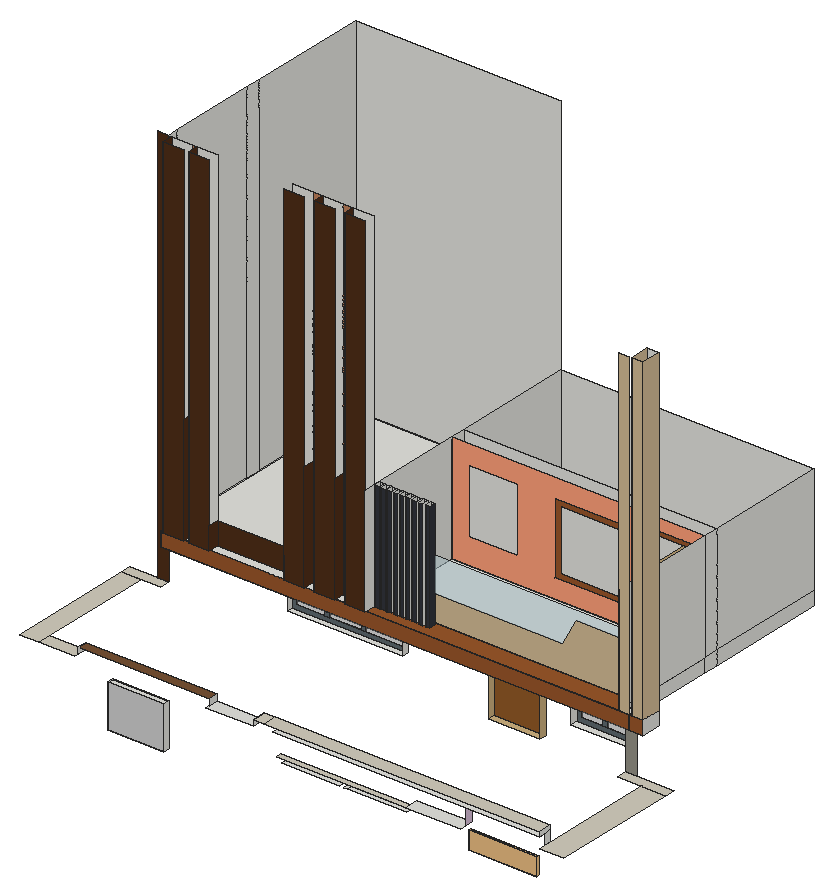
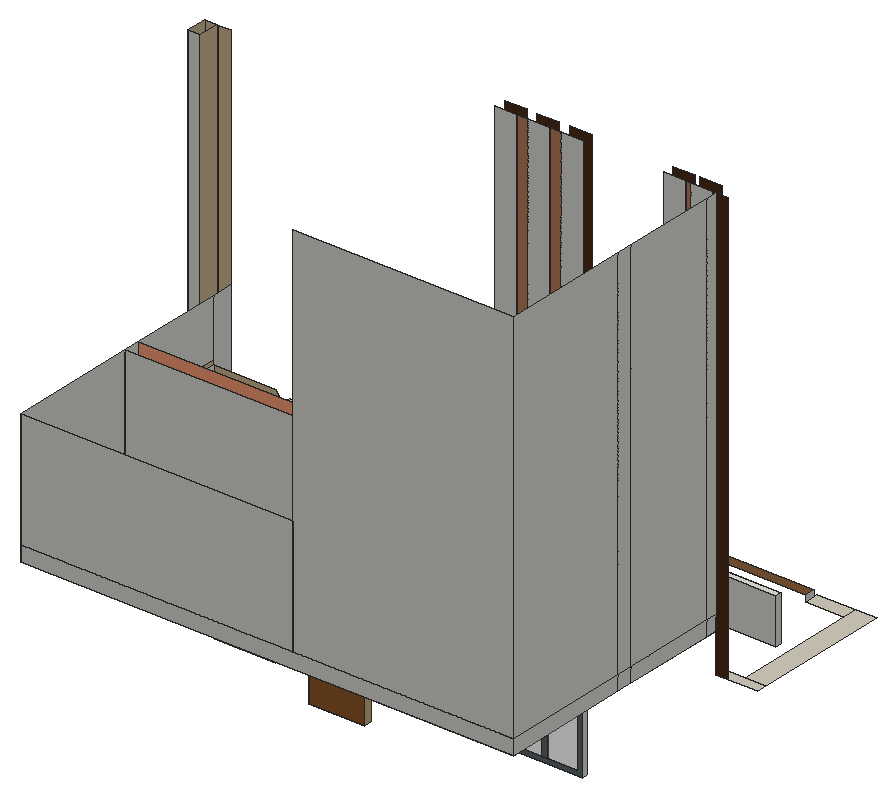
# SketchUp Ruby script. Lengths in inches.
U = 1.inch
M = Sketchup.active_model
def pt(a) = Geom::Point3d.new(a.map { |v| v * U })
def face(e, loops, mat)
  f = e.add_face(loops[0].map { |a| pt(a) })
  loops[1..].each { |l| e.add_face(l.map { |a| pt(a) }).erase! }
  f.material = f.back_material = mat if mat
  f
end
# faces: each face lists its corners as indices into pts; further lists are holes
def faces(e, pts, list, mat = nil) = list.each { |f| face(e, (f[0].is_a?(Array) ? f : [f]).map { |l| l.map { |i| pts[i] } }, mat) }
# xy, xz, yz: faces in a plane at the given z, y or x. An outline is a flat list of corners, or four numbers for a rectangle; further outlines are holes
def ring(l) = l.size == 4 ? [[l[0], l[1]], [l[2], l[1]], [l[2], l[3]], [l[0], l[3]]] : l.each_slice(2).to_a
def flat(e, list, mat, &to3) = list.each { |f| face(e, (f[0].is_a?(Array) ? f : [f]).map { |l| ring(l).map { |u, v| to3.(u, v) } }, mat) }
def xy(e, z, list, mat = nil) = flat(e, list, mat) { |x, y| [x, y, z] }
def xz(e, y, list, mat = nil) = flat(e, list, mat) { |x, z| [x, y, z] }
def yz(e, x, list, mat = nil) = flat(e, list, mat) { |y, z| [x, y, z] }
def lines(e, pts, list) = list.each { |a, b| e.add_line(pt(pts[a]), pt(pts[b])) }
# prism: a flat outline (further loops are holes) pulled along v
def prism(e, loops, v, mat = nil)
  f = face(e, loops, mat); d = Geom::Vector3d.new(v.map { |x| x * U })
  f.pushpull(f.normal.samedirection?(d) ? d.length : -d.length)
end
def box(e, o, s, mat = nil) = prism(e, [[o, [o[0] + s[0], o[1], o[2]], [o[0] + s[0], o[1] + s[1], o[2]], [o[0], o[1] + s[1], o[2]]]], [0, 0, s[2]], mat)
def at(x, y, z, deg = 0) = Geom::Transformation.translation(pt([x, y, z])) * Geom::Transformation.rotation(ORIGIN, Z_AXIS, deg.degrees)
def axes(o, x, y, z) = Geom::Transformation.new([*x, 0, *y, 0, *z, 0, *pt(o).to_a, 1])
def part(name) = M.definitions.add(name)
# library, detail: a bought-in or finely detailed component or shape, given as its bounding box
def library(name, o, s) = part(name).tap { |d| box(d.entities, o, s) }
def detail(e, o, s) = box(e.add_group.entities, o, s)
def put(e, d, t, mat = nil) = e.add_instance(d, t).tap { |i| i.material = mat if mat }
def group(e, t, mat = nil) = e.add_group.tap { |g| g.transformation = t; g.material = mat if mat }.entities
root = M.entities
M.materials.add("[0026_LightSalmon]").color = [255, 160, 122]
M.materials.add("[0046_Gold]").color = [226, 191, 0]
M.materials.add("[0118_Thistle]").color = [216, 191, 216]
M.materials.add("[Carrera Marble]").color = [207, 207, 207]
M.materials.add("[Formica Beige]").color = [211, 187, 149]
M.materials.add("[Formica Graystone]").color = [209, 204, 189]
M.materials.add("[Formica Graystone]1").color = [149, 146, 135]
M.materials.add("[Formica Laminate Dark]").color = [50, 53, 60]
M.materials.add("[Formica Speckled Grey]").color = [94, 105, 111]
M.materials.add("[Sandstone]").color = [118, 81, 52]
M.materials.add("[Translucent Glass Gray]").color = [128, 128, 128]
M.materials["[Translucent Glass Gray]"].alpha = 0.5
M.materials.add("[Translucent Glass Safety]").color = [204, 235, 244]
M.materials["[Translucent Glass Safety]"].alpha = 0.5
M.materials.add("[Wood Cherry Original]").color = [152, 86, 42]
M.materials.add("[Wood Floor Light]").color = [204, 176, 127]
M.materials.add("[Wood Floor Parquet]").color = [145, 89, 39]
M.materials.add("[Wood Veneer 01]").color = [79, 46, 24]
M.materials.add("[Wood Veneer 02]").color = [190, 128, 91]
c1 = library("Shloka",[1.82,0,0],[112.97,25.6,12])
xy(root,17.66,[[410.04,348.07,486.1,358.26]],"[Wood Floor Light]")
xy(root,51.82,[[530.86,348.07,613.92,359.32]])
xy(root,56.31,[[116.08,348.07,284.86,355.95]])
xy(root,58.17,[[130.9,0,212.59,8.25]])
xy(root,96.37,[[[377.34,9.54,462.5,17.41],[458.64,12.51,458.96,12.55,459.26,12.67,459.52,12.875,459.72,13.13,459.85,13.43,459.89,13.76,459.85,14.08,459.72,14.38,459.52,14.64,459.26,14.84,458.96,14.96,458.64,15.01,458.32,14.96,458.01,14.84,457.76,14.64,457.56,14.38,457.43,14.08,457.39,13.76,457.43,13.43,457.56,13.13,457.76,12.875,458.01,12.67,458.32,12.55],[453.95,12.51,454.28,12.55,454.58,12.67,454.84,12.875,455.03,13.13,455.16,13.43,455.2,13.76,455.16,14.08,455.03,14.38,454.84,14.64,454.58,14.84,454.28,14.96,453.95,15.01,453.63,14.96,453.33,14.84,453.07,14.64,452.87,14.38,452.74,14.08,452.7,13.76,452.74,13.43,452.87,13.13,453.07,12.875,453.33,12.67,453.63,12.55],[448.45,12.51,448.78,12.55,449.08,12.67,449.34,12.875,449.53,13.13,449.66,13.43,449.7,13.76,449.66,14.08,449.53,14.38,449.34,14.64,449.08,14.84,448.78,14.96,448.45,15.01,448.13,14.96,447.83,14.84,447.57,14.64,447.37,14.38,447.24,14.08,447.2,13.76,447.24,13.43,447.37,13.13,447.57,12.875,447.83,12.67,448.13,12.55],[442.45,12.51,442.78,12.55,443.08,12.67,443.34,12.875,443.53,13.13,443.66,13.43,443.7,13.76,443.66,14.08,443.53,14.38,443.34,14.64,443.08,14.84,442.78,14.96,442.45,15.01,442.13,14.96,441.83,14.84,441.57,14.64,441.37,14.38,441.24,14.08,441.2,13.76,441.24,13.43,441.37,13.13,441.57,12.875,441.83,12.67,442.13,12.55],[436.2,12.51,436.53,12.55,436.83,12.67,437.09,12.875,437.28,13.13,437.41,13.43,437.45,13.76,437.41,14.08,437.28,14.38,437.09,14.64,436.83,14.84,436.53,14.96,436.2,15.01,435.88,14.96,435.58,14.84,435.32,14.64,435.12,14.38,434.99,14.08,434.95,13.76,434.99,13.43,435.12,13.13,435.32,12.875,435.58,12.67,435.88,12.55],[430.51,12.51,430.84,12.55,431.14,12.67,431.4,12.875,431.6,13.13,431.72,13.43,431.76,13.76,431.72,14.08,431.6,14.38,431.4,14.64,431.14,14.84,430.84,14.96,430.51,15.01,430.19,14.96,429.89,14.84,429.63,14.64,429.43,14.38,429.31,14.08,429.26,13.76,429.31,13.43,429.43,13.13,429.63,12.875,429.89,12.67,430.19,12.55],[424.64,12.51,424.96,12.55,425.26,12.67,425.52,12.875,425.72,13.13,425.85,13.43,425.89,13.76,425.85,14.08,425.72,14.38,425.52,14.64,425.26,14.84,424.96,14.96,424.64,15.01,424.32,14.96,424.01,14.84,423.76,14.64,423.56,14.38,423.43,14.08,423.39,13.76,423.43,13.43,423.56,13.13,423.76,12.875,424.01,12.67,424.32,12.55],[418.89,12.51,419.21,12.55,419.51,12.67,419.77,12.875,419.97,13.13,420.1,13.43,420.14,13.76,420.1,14.08,419.97,14.38,419.77,14.64,419.51,14.84,419.21,14.96,418.89,15.01,418.57,14.96,418.26,14.84,418.01,14.64,417.81,14.38,417.68,14.08,417.64,13.76,417.68,13.43,417.81,13.13,418.01,12.875,418.26,12.67,418.57,12.55],[414.01,12.51,414.34,12.55,414.64,12.67,414.9,12.875,415.1,13.13,415.22,13.43,415.26,13.76,415.22,14.08,415.1,14.38,414.9,14.64,414.64,14.84,414.34,14.96,414.01,15.01,413.69,14.96,413.39,14.84,413.13,14.64,412.93,14.38,412.81,14.08,412.76,13.76,412.81,13.43,412.93,13.13,413.13,12.875,413.39,12.67,413.69,12.55],[408.45,12.51,408.78,12.55,409.08,12.67,409.34,12.875,409.53,13.13,409.66,13.43,409.7,13.76,409.66,14.08,409.53,14.38,409.34,14.64,409.08,14.84,408.78,14.96,408.45,15.01,408.13,14.96,407.83,14.84,407.57,14.64,407.37,14.38,407.24,14.08,407.2,13.76,407.24,13.43,407.37,13.13,407.57,12.875,407.83,12.67,408.13,12.55],[402.58,12.51,402.9,12.55,403.2,12.67,403.46,12.875,403.66,13.13,403.78,13.43,403.83,13.76,403.78,14.08,403.66,14.38,403.46,14.64,403.2,14.84,402.9,14.96,402.58,15.01,402.25,14.96,401.95,14.84,401.69,14.64,401.49,14.38,401.37,14.08,401.33,13.76,401.37,13.43,401.49,13.13,401.69,12.875,401.95,12.67,402.25,12.55],[396.95,12.51,397.28,12.55,397.58,12.67,397.84,12.875,398.03,13.13,398.16,13.43,398.2,13.76,398.16,14.08,398.03,14.38,397.84,14.64,397.58,14.84,397.28,14.96,396.95,15.01,396.63,14.96,396.33,14.84,396.07,14.64,395.87,14.38,395.74,14.08,395.7,13.76,395.74,13.43,395.87,13.13,396.07,12.875,396.33,12.67,396.63,12.55],[390.45,12.51,390.78,12.55,391.08,12.67,391.34,12.875,391.53,13.13,391.66,13.43,391.7,13.76,391.66,14.08,391.53,14.38,391.34,14.64,391.08,14.84,390.78,14.96,390.45,15.01,390.13,14.96,389.83,14.84,389.57,14.64,389.37,14.38,389.24,14.08,389.2,13.76,389.24,13.43,389.37,13.13,389.57,12.875,389.83,12.67,390.13,12.55],[384.7,12.51,385.03,12.55,385.33,12.67,385.59,12.875,385.78,13.13,385.91,13.43,385.95,13.76,385.91,14.08,385.78,14.38,385.59,14.64,385.33,14.84,385.03,14.96,384.7,15.01,384.38,14.96,384.08,14.84,383.82,14.64,383.62,14.38,383.49,14.08,383.45,13.76,383.49,13.43,383.62,13.13,383.82,12.875,384.08,12.67,384.38,12.55],[380.14,12.51,380.47,12.55,380.77,12.67,381.03,12.875,381.23,13.13,381.35,13.43,381.39,13.76,381.35,14.08,381.23,14.38,381.03,14.64,380.77,14.84,380.47,14.96,380.14,15.01,379.82,14.96,379.52,14.84,379.26,14.64,379.06,14.38,378.94,14.08,378.89,13.76,378.94,13.43,379.06,13.13,379.26,12.875,379.52,12.67,379.82,12.55]],[468.46,9.54,474.42,17.41],[[474.42,9.54,560.77,17.41],[555.89,12.51,556.21,12.55,556.51,12.67,556.77,12.875,556.97,13.13,557.1,13.43,557.14,13.76,557.1,14.08,556.97,14.38,556.77,14.64,556.51,14.84,556.21,14.96,555.89,15.01,555.57,14.96,555.26,14.84,555.01,14.64,554.81,14.38,554.68,14.08,554.64,13.76,554.68,13.43,554.81,13.13,555.01,12.875,555.26,12.67,555.57,12.55],[550.39,12.51,550.71,12.55,551.01,12.67,551.27,12.875,551.47,13.13,551.6,13.43,551.64,13.76,551.6,14.08,551.47,14.38,551.27,14.64,551.01,14.84,550.71,14.96,550.39,15.01,550.07,14.96,549.76,14.84,549.51,14.64,549.31,14.38,549.18,14.08,549.14,13.76,549.18,13.43,549.31,13.13,549.51,12.875,549.76,12.67,550.07,12.55],[544.76,12.51,545.09,12.55,545.39,12.67,545.65,12.875,545.85,13.13,545.97,13.43,546.01,13.76,545.97,14.08,545.85,14.38,545.65,14.64,545.39,14.84,545.09,14.96,544.76,15.01,544.44,14.96,544.14,14.84,543.88,14.64,543.68,14.38,543.56,14.08,543.51,13.76,543.56,13.43,543.68,13.13,543.88,12.875,544.14,12.67,544.44,12.55],[539.51,12.51,539.84,12.55,540.14,12.67,540.4,12.875,540.6,13.13,540.72,13.43,540.76,13.76,540.72,14.08,540.6,14.38,540.4,14.64,540.14,14.84,539.84,14.96,539.51,15.01,539.19,14.96,538.89,14.84,538.63,14.64,538.43,14.38,538.31,14.08,538.26,13.76,538.31,13.43,538.43,13.13,538.63,12.875,538.89,12.67,539.19,12.55],[533.7,12.51,534.03,12.55,534.33,12.67,534.59,12.875,534.78,13.13,534.91,13.43,534.95,13.76,534.91,14.08,534.78,14.38,534.59,14.64,534.33,14.84,534.03,14.96,533.7,15.01,533.38,14.96,533.08,14.84,532.82,14.64,532.62,14.38,532.49,14.08,532.45,13.76,532.49,13.43,532.62,13.13,532.82,12.875,533.08,12.67,533.38,12.55],[528.2,12.51,528.53,12.55,528.83,12.67,529.09,12.875,529.28,13.13,529.41,13.43,529.45,13.76,529.41,14.08,529.28,14.38,529.09,14.64,528.83,14.84,528.53,14.96,528.2,15.01,527.88,14.96,527.58,14.84,527.32,14.64,527.12,14.38,526.99,14.08,526.95,13.76,526.99,13.43,527.12,13.13,527.32,12.875,527.58,12.67,527.88,12.55],[522.33,12.51,522.65,12.55,522.95,12.67,523.21,12.875,523.41,13.13,523.53,13.43,523.58,13.76,523.53,14.08,523.41,14.38,523.21,14.64,522.95,14.84,522.65,14.96,522.33,15.01,522,14.96,521.7,14.84,521.44,14.64,521.24,14.38,521.12,14.08,521.08,13.76,521.12,13.43,521.24,13.13,521.44,12.875,521.7,12.67,522,12.55],[517.01,12.51,517.34,12.55,517.64,12.67,517.9,12.875,518.1,13.13,518.22,13.43,518.26,13.76,518.22,14.08,518.1,14.38,517.9,14.64,517.64,14.84,517.34,14.96,517.01,15.01,516.69,14.96,516.39,14.84,516.13,14.64,515.93,14.38,515.81,14.08,515.76,13.76,515.81,13.43,515.93,13.13,516.13,12.875,516.39,12.67,516.69,12.55],[511.7,12.51,512.03,12.55,512.33,12.67,512.59,12.875,512.78,13.13,512.91,13.43,512.95,13.76,512.91,14.08,512.78,14.38,512.59,14.64,512.33,14.84,512.03,14.96,511.7,15.01,511.38,14.96,511.08,14.84,510.82,14.64,510.62,14.38,510.49,14.08,510.45,13.76,510.49,13.43,510.62,13.13,510.82,12.875,511.08,12.67,511.38,12.55],[506.08,12.51,506.4,12.55,506.7,12.67,506.96,12.875,507.16,13.13,507.28,13.43,507.33,13.76,507.28,14.08,507.16,14.38,506.96,14.64,506.7,14.84,506.4,14.96,506.08,15.01,505.75,14.96,505.45,14.84,505.19,14.64,504.99,14.38,504.87,14.08,504.83,13.76,504.87,13.43,504.99,13.13,505.19,12.875,505.45,12.67,505.75,12.55],[500.95,12.51,501.28,12.55,501.58,12.67,501.84,12.875,502.03,13.13,502.16,13.43,502.2,13.76,502.16,14.08,502.03,14.38,501.84,14.64,501.58,14.84,501.28,14.96,500.95,15.01,500.63,14.96,500.33,14.84,500.07,14.64,499.87,14.38,499.74,14.08,499.7,13.76,499.74,13.43,499.87,13.13,500.07,12.875,500.33,12.67,500.63,12.55],[495.14,12.51,495.46,12.55,495.76,12.67,496.02,12.875,496.22,13.13,496.35,13.43,496.39,13.76,496.35,14.08,496.22,14.38,496.02,14.64,495.76,14.84,495.46,14.96,495.14,15.01,494.82,14.96,494.51,14.84,494.26,14.64,494.06,14.38,493.93,14.08,493.89,13.76,493.93,13.43,494.06,13.13,494.26,12.875,494.51,12.67,494.82,12.55],[489.83,12.51,490.15,12.55,490.45,12.67,490.71,12.875,490.91,13.13,491.03,13.43,491.08,13.76,491.03,14.08,490.91,14.38,490.71,14.64,490.45,14.84,490.15,14.96,489.83,15.01,489.5,14.96,489.2,14.84,488.94,14.64,488.74,14.38,488.62,14.08,488.58,13.76,488.62,13.43,488.74,13.13,488.94,12.875,489.2,12.67,489.5,12.55],[484.01,12.51,484.34,12.55,484.64,12.67,484.9,12.875,485.1,13.13,485.22,13.43,485.26,13.76,485.22,14.08,485.1,14.38,484.9,14.64,484.64,14.84,484.34,14.96,484.01,15.01,483.69,14.96,483.39,14.84,483.13,14.64,482.93,14.38,482.81,14.08,482.76,13.76,482.81,13.43,482.93,13.13,483.13,12.875,483.39,12.67,483.69,12.55],[478.45,12.51,478.78,12.55,479.08,12.67,479.34,12.875,479.53,13.13,479.66,13.43,479.7,13.76,479.66,14.08,479.53,14.38,479.34,14.64,479.08,14.84,478.78,14.96,478.45,15.01,478.13,14.96,477.83,14.84,477.57,14.64,477.37,14.38,477.24,14.08,477.2,13.76,477.24,13.43,477.37,13.13,477.57,12.875,477.83,12.67,478.13,12.55]]])
xy(root,102.25,[[370.65,9.54,560.77,17.41],[560.77,9.54,566.39,17.41]],"[Formica Graystone]")
xy(root,108,[[566.39,1.67,646.62,21.38]])
xy(root,120.61,[[130.9,0,212.59,8.25]])
xy(root,122.6875,[[762.14,1.67,797.12,189.01],[727.17,189.01,797.12,203.79]],"[Formica Graystone]")
xy(root,136.125,[[273.1875,1.67,342.51,21.38]])
xy(root,136.125,[[0,1.67,28.1,189.01],[28.1,1.67,80.35,21.38],[0,189.01,56.2,203.79]],"[Formica Graystone]")
xy(root,138.11,[[370.65,1.67,370.65,21.38,646.62,21.38,646.62,11.52,762.14,11.52,762.14,1.67]])
xy(root,145.125,[[342.51,1.67,357.9375,21.38],[357.9375,1.67,762.14,21.38]],"[Formica Graystone]")
xy(root,145.125,[[80.35,8.25,273.1875,21.38]],"[Sandstone]")
xy(root,151.43,[[410.04,348.07,486.1,358.26]],"[Wood Floor Light]")
xy(root,160.38,[[530.86,348.07,613.92,359.32]])
xy(root,160.63,[[116.08,348.07,284.86,355.95]])
xy(root,189,[[56.2,190.11,56.2,348.07,727.17,348.07,727.17,203.79,742.93,203.79,742.93,190.11],[742.93,190.11,763.24,218.11],[56.2,348.07,727.17,370.07],[56.2,370.07,727.17,548.03]])
xy(root,209.5,[[61.07,188.11,91,190.11],[98.07,188.11,128,190.11],[238.01,188.11,267.9375,190.11],[282.39,188.11,312.3125,190.11],[326.76,188.11,356.6875,190.11],
  [56.2,190.11,61.07,203.79],[61.07,190.11,91,203.79],[91,190.11,98.07,203.79],[98.07,190.11,128,203.79],[128,190.11,238.01,203.79],
  [238.01,190.11,267.9375,203.79],[267.9375,190.11,282.39,203.79],[282.39,190.11,312.3125,203.79],[312.3125,190.11,326.76,203.79],[326.76,190.11,356.6875,203.79],
  [727.17,190.11,742.93,203.79],[742.93,190.11,746.31,203.79],[746.31,190.11,763.24,218.11],[56.2,203.79,356.6875,548.03],[742.93,203.79,746.31,218.11],
  [358.51,205,364.9375,214.21],[367.14,205,373.5625,214.21],[376.01,205,382.4375,214.21],[385.08,205,391.5,214.21],[393.95,205,400.375,214.21],
  [403.08,205,409.5,214.21],[412.39,205,418.8125,214.21],[422.26,205,428.6875,214.21],[432.2,205,438.625,214.21],[356.6875,219.56,727.17,237.64],
  [356.6875,237.64,727.17,348.07],[356.6875,348.07,727.17,370.07],[356.6875,370.07,727.17,548.03]])
xy(root,209.5,[[[356.6875,190.11,727.17,219.56],[358.51,205,364.9375,214.21],[367.14,205,373.5625,214.21],[376.01,205,382.4375,214.21],[385.08,205,391.5,214.21],[393.95,205,400.375,214.21],[403.08,205,409.5,214.21],[412.39,205,418.8125,214.21],[422.26,205,428.6875,214.21],[432.2,205,438.625,214.21]]],"[Wood Cherry Original]")
xz(root,0,[[130.9,58.17,212.59,120.61]],"[Carrera Marble]")
xz(root,8.25,[[130.9,58.17,212.59,120.61]])
xz(root,188.11,[[61.07,209.5,91,723.1875],[98.07,209.5,128,723.1875],[238.01,209.5,267.9375,723.1875],[282.39,209.5,312.3125,723.1875],[326.76,209.5,356.6875,723.1875]],"[Wood Veneer 01]")
xz(root,190.11,[[727.17,209.5,742.93,679.64],[746.31,209.5,763.24,679.64]],"[Formica Beige]")
xz(root,190.11,[[56.2,189,742.93,209.5],[742.93,189,763.24,209.5]],"[Wood Cherry Original]")
xz(root,203.79,[[727.17,189,742.93,209.5],[61.07,209.5,91,723.1875],[98.07,209.5,128,723.1875],[238.01,209.5,267.9375,723.1875],[282.39,209.5,312.3125,723.1875],
  [326.76,209.5,356.6875,723.1875]])
xz(root,203.79,[[727.17,122.6875,742.93,189]],"[Formica Graystone]1")
xz(root,203.79,[[40.4375,136.125,56.2,723.1875],[56.2,209.5,61.07,723.1875],[128,209.5,238.01,242.08]],"[Wood Veneer 01]")
xz(root,203.79,[[91,209.5,98.07,723.1875],[267.9375,209.5,282.39,723.1875],[312.3125,209.5,326.76,723.1875]],"[Wood Veneer 02]")
xz(root,205,[[358.51,209.5,364.9375,369],[367.14,209.5,373.5625,369],[376.01,209.5,382.4375,369],[385.08,209.5,391.5,369],[393.95,209.5,400.375,369],
  [403.08,209.5,409.5,369],[412.39,209.5,418.8125,369],[422.26,209.5,428.6875,369],[432.2,209.5,438.625,369]],"[Formica Laminate Dark]")
xz(root,214.21,[[358.51,209.5,364.9375,369],[367.14,209.5,373.5625,369],[376.01,209.5,382.4375,369],[385.08,209.5,391.5,369],[393.95,209.5,400.375,369],
  [403.08,209.5,409.5,369],[412.39,209.5,418.8125,369],[422.26,209.5,428.6875,369],[432.2,209.5,438.625,369]])
xz(root,218.11,[[742.93,189,763.24,209.5],[746.31,209.5,763.24,679.64]])
xz(root,219.56,[[356.6875,209.5,727.17,209.5,727.17,284.4375,641.9,284.4375,640.93,282.64,621.625,246.97,356.6875,246.97]],"[Formica Beige]")
xz(root,237.64,[[356.6875,209.5,727.17,284.4375]],"[Translucent Glass Safety]")
xz(root,348.07,[[[356.6875,209.5,636.95,209.5,636.95,351.5625,715.32,351.5625,715.32,209.5,727.17,209.5,727.17,369,356.6875,369],[507.59,236.79,612.84,342.04],[380.95,246.23,452.45,341.42]]],"[0026_LightSalmon]")
xz(root,348.07,[[[636.95,209.5,715.32,351.5625],[642.89,215.44,709.38,345.62]],[[507.59,236.79,612.84,342.04],[515.72,244.91,604.72,333.92]]],"[Wood Cherry Original]")
xz(root,348.07,[[[642.89,215.44,709.38,215.44,709.38,345.62,696.74,345.62,642.89,296.77],[649.28,265.99,653.91,288.67]]],"[Wood Floor Light]")
xz(root,355.95,[[[116.08,56.31,284.86,160.63],[122.64,62.88,278.29,154.0625]],[163.73,62.88,170.86,154.0625],[217.45,62.88,224.57,154.0625]],"[Formica Speckled Grey]")
xz(root,355.95,[[122.64,62.88,163.73,154.0625],[170.86,62.88,217.45,154.0625],[224.57,62.88,278.29,154.0625]],"[Translucent Glass Gray]")
xz(root,358.26,[[410.04,17.66,486.1,151.43]],"[Wood Floor Parquet]")
xz(root,359.32,[[[530.86,51.82,613.92,160.38],[537.58,58.53,607.21,153.66]],[568.49,58.53,575.72,153.66]],"[Formica Speckled Grey]")
xz(root,359.32,[[537.58,58.53,568.49,153.66],[575.72,58.53,607.21,153.66]],"[Translucent Glass Gray]")
xz(root,370.07,[[356.6875,209.5,727.17,369]])
xz(root,548.03,[[56.2,189,727.17,209.5],[56.2,209.5,356.6875,723.1875],[356.6875,209.5,727.17,369]])
yz(root,56.2,[[190.11,189,203.79,209.5],[203.79,189,219.56,209.5],[219.56,189,348.07,209.5],[348.07,189,370.07,209.5],[370.07,189,548.03,209.5],
  [203.79,209.5,219.56,723.1875],[219.56,209.5,348.07,723.1875],[348.07,209.5,370.07,723.1875],[370.07,209.5,548.03,723.1875]])
yz(root,61.07,[[188.11,209.5,203.79,723.1875]],"[Wood Veneer 01]")
yz(root,80.35,[[8.25,136.125,21.38,145.125]])
yz(root,91,[[188.11,209.5,203.79,369]],"[Wood Veneer 01]")
yz(root,98.07,[[188.11,209.5,203.79,723.1875]],"[Wood Veneer 01]")
yz(root,116.08,[[348.07,56.31,355.95,160.63]])
yz(root,128,[[188.11,209.5,203.79,242.08]],"[Wood Veneer 01]")
yz(root,130.9,[[0,58.17,8.25,120.61]])
yz(root,212.59,[[0,58.17,8.25,120.61]])
yz(root,238.01,[[188.11,209.5,203.79,242.08]],"[Wood Veneer 01]")
yz(root,267.9375,[[188.11,209.5,203.79,369]],"[Wood Veneer 01]")
yz(root,273.1875,[[8.25,136.125,21.38,145.125]])
yz(root,282.39,[[188.11,209.5,203.79,723.1875]],"[Wood Veneer 01]")
yz(root,284.86,[[348.07,56.31,355.95,160.63]])
yz(root,312.3125,[[188.11,209.5,203.79,369]],"[Wood Veneer 01]")
yz(root,326.76,[[188.11,209.5,203.79,723.1875]],"[Wood Veneer 01]")
yz(root,342.51,[[1.67,136.125,21.38,145.125]])
yz(root,356.6875,[[188.11,209.5,203.79,369],[[203.79,209.5,219.56,209.5,219.56,246.97,216.87,246.97,216.87,255.23,219.56,255.23,219.56,284.4375,237.64,284.4375,237.64,209.5,348.07,209.5,348.07,369,203.79,369],[227.13,285.1,226.4,285.19,225.72,285.47,225.14,285.92,224.69,286.5,224.41,287.18,224.32,287.91,224.41,288.64,224.69,289.32,225.14,289.9,225.72,290.35,226.4,290.625,227.13,290.72,227.86,290.625,228.54,290.35,229.12,289.9,229.57,289.32,229.85,288.64,229.94,287.91,229.85,287.18,229.57,286.5,229.12,285.92,228.54,285.47,227.86,285.19]],[219.56,209.5,237.64,284.4375],[348.07,209.5,370.07,369],[370.07,209.5,548.03,369]])
yz(root,358.51,[[205,209.5,214.21,369]])
yz(root,364.9375,[[205,209.5,214.21,369]])
yz(root,367.14,[[205,209.5,214.21,369]])
yz(root,373.5625,[[205,209.5,214.21,369]])
yz(root,376.01,[[205,209.5,214.21,369]])
yz(root,382.4375,[[205,209.5,214.21,369]])
yz(root,385.08,[[205,209.5,214.21,369]])
yz(root,391.5,[[205,209.5,214.21,369]])
yz(root,393.95,[[205,209.5,214.21,369]])
yz(root,400.375,[[205,209.5,214.21,369]])
yz(root,403.08,[[205,209.5,214.21,369]])
yz(root,409.5,[[205,209.5,214.21,369]])
yz(root,410.04,[[348.07,17.66,358.26,151.43]],"[Wood Floor Light]")
yz(root,412.39,[[205,209.5,214.21,369]])
yz(root,418.8125,[[205,209.5,214.21,369]])
yz(root,422.26,[[205,209.5,214.21,369]])
yz(root,428.6875,[[205,209.5,214.21,369]])
yz(root,432.2,[[205,209.5,214.21,369]])
yz(root,438.625,[[205,209.5,214.21,369]],"[Formica Laminate Dark]")
yz(root,486.1,[[348.07,17.66,358.26,151.43]],"[Wood Floor Light]")
yz(root,530.86,[[348.07,51.82,359.32,160.38]])
yz(root,613.92,[[348.07,51.82,359.32,160.38]])
yz(root,646.62,[[11.52,108,21.38,138.11]],"[0118_Thistle]")
yz(root,727.17,[[203.79,189,219.56,209.5],[219.56,189,348.07,209.5],[348.07,189,370.07,209.5],[370.07,189,548.03,209.5],[190.11,209.5,219.56,369],
  [219.56,209.5,237.64,284.4375],[237.64,209.5,237.64,291.5,219.56,291.5,219.56,369,348.07,369,348.07,209.5],[348.07,209.5,370.07,369],[370.07,209.5,548.03,369]])
yz(root,742.93,[[190.11,189,203.79,209.5],[203.79,189,218.11,209.5]])
yz(root,746.31,[[190.11,209.5,218.11,679.64]],"[Formica Beige]")
yz(root,762.14,[[11.52,122.6875,21.38,138.11],[1.67,138.11,21.38,145.125]])
yz(root,763.24,[[190.11,189,218.11,209.5]])
yz(root,763.24,[[190.11,209.5,218.11,679.64]],"[Formica Beige]")
put(root,c1,axes([652.52,11.52,80.53],[0.88,0,0],[0,0,1],[0,-0.31,0]),"[0046_Gold]")
